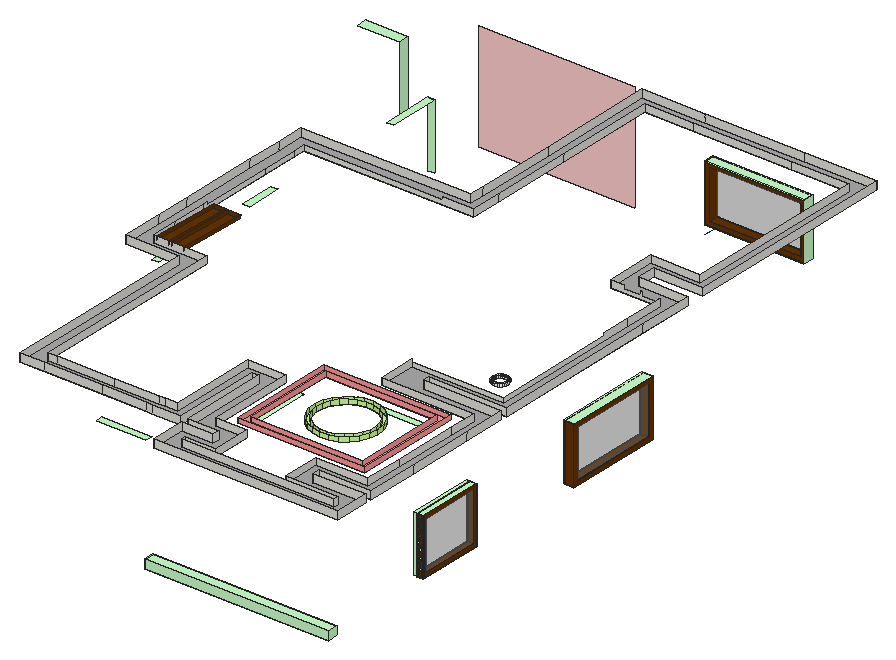
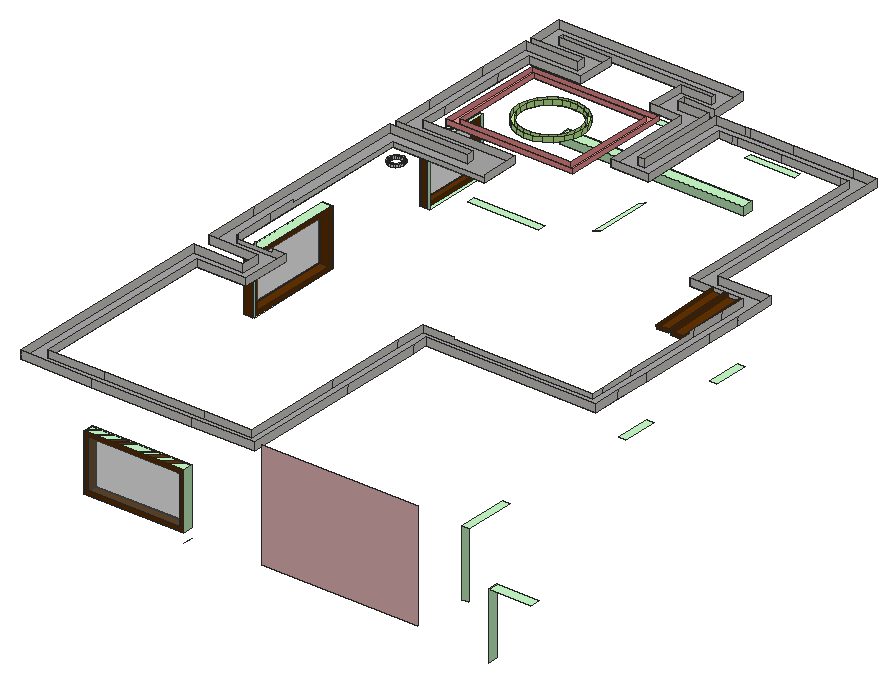
# SketchUp Ruby script. Lengths in inches.
U = 1.inch
M = Sketchup.active_model
def pt(a) = Geom::Point3d.new(a.map { |v| v * U })
def face(e, loops, mat)
  f = e.add_face(loops[0].map { |a| pt(a) })
  loops[1..].each { |l| e.add_face(l.map { |a| pt(a) }).erase! }
  f.material = f.back_material = mat if mat
  f
end
# faces: each face lists its corners as indices into pts; further lists are holes
def faces(e, pts, list, mat = nil) = list.each { |f| face(e, (f[0].is_a?(Array) ? f : [f]).map { |l| l.map { |i| pts[i] } }, mat) }
# xy, xz, yz: faces in a plane at the given z, y or x. An outline is a flat list of corners, or four numbers for a rectangle; further outlines are holes
def ring(l) = l.size == 4 ? [[l[0], l[1]], [l[2], l[1]], [l[2], l[3]], [l[0], l[3]]] : l.each_slice(2).to_a
def flat(e, list, mat, &to3) = list.each { |f| face(e, (f[0].is_a?(Array) ? f : [f]).map { |l| ring(l).map { |u, v| to3.(u, v) } }, mat) }
def xy(e, z, list, mat = nil) = flat(e, list, mat) { |x, y| [x, y, z] }
def xz(e, y, list, mat = nil) = flat(e, list, mat) { |x, z| [x, y, z] }
def yz(e, x, list, mat = nil) = flat(e, list, mat) { |y, z| [x, y, z] }
def lines(e, pts, list) = list.each { |a, b| e.add_line(pt(pts[a]), pt(pts[b])) }
# prism: a flat outline (further loops are holes) pulled along v
def prism(e, loops, v, mat = nil)
  f = face(e, loops, mat); d = Geom::Vector3d.new(v.map { |x| x * U })
  f.pushpull(f.normal.samedirection?(d) ? d.length : -d.length)
end
def box(e, o, s, mat = nil) = prism(e, [[o, [o[0] + s[0], o[1], o[2]], [o[0] + s[0], o[1] + s[1], o[2]], [o[0], o[1] + s[1], o[2]]]], [0, 0, s[2]], mat)
def at(x, y, z, deg = 0) = Geom::Transformation.translation(pt([x, y, z])) * Geom::Transformation.rotation(ORIGIN, Z_AXIS, deg.degrees)
def axes(o, x, y, z) = Geom::Transformation.new([*x, 0, *y, 0, *z, 0, *pt(o).to_a, 1])
def part(name) = M.definitions.add(name)
# library, detail: a bought-in or finely detailed component or shape, given as its bounding box
def library(name, o, s) = part(name).tap { |d| box(d.entities, o, s) }
def detail(e, o, s) = box(e.add_group.entities, o, s)
def put(e, d, t, mat = nil) = e.add_instance(d, t).tap { |i| i.material = mat if mat }
def group(e, t, mat = nil) = e.add_group.tap { |g| g.transformation = t; g.material = mat if mat }.entities
root = M.entities
M.materials.add("[Color A01]").color = [255, 204, 204]
M.materials.add("[Color A02]").color = [255, 153, 153]
M.materials.add("[Color C08]").color = [102, 51, 0]
M.materials.add("[Color F02]").color = [204, 255, 153]
M.materials.add("[Color G01]").color = [204, 255, 204]
M.materials.add("[Color M00]").color = [255, 255, 255]
M.materials.add("[Color M03]").color = [170, 170, 170]
M.materials.add("[Marble Carrara Gold Floor Tile]").color = [225, 223, 217]
M.materials.add("[Translucent Glass Gray]").color = [128, 128, 128]
M.materials["[Translucent Glass Gray]"].alpha = 0.5
c1 = part("Group\#14")
xy(c1.entities,0,[[0,0,8.11,83.5625]])
xy(c1.entities,3.3125,[[7.9,3.57,8.11,80]])
xy(c1.entities,3.3125,[[0,3.57,7.9,80]],"[Color C08]")
xy(c1.entities,44.6875,[[0,3.57,7.9,80],[7.9,3.57,8.11,80]])
xy(c1.entities,48,[[0,0,8.11,83.5625]],"[Color C08]")
xz(c1.entities,0,[[0,0,8.11,48]],"[Color C08]")
xz(c1.entities,3.57,[[7.9,3.3125,8.11,44.6875]])
xz(c1.entities,3.57,[[0,3.3125,7.9,44.6875]],"[Color C08]")
xz(c1.entities,80,[[7.9,3.3125,8.11,44.6875]])
xz(c1.entities,80,[[0,3.3125,7.9,44.6875]],"[Color C08]")
xz(c1.entities,83.5625,[[0,0,8.11,48]],"[Color C08]")
yz(c1.entities,0,[[[0,0,83.5625,48],[3.57,3.3125,80,44.6875]]],"[Color C08]")
yz(c1.entities,7.9,[[3.57,3.3125,80,44.6875]],"[Translucent Glass Gray]")
yz(c1.entities,8.11,[[[0,0,83.5625,48],[3.57,3.3125,80,44.6875]]],"[Color C08]")
box(root,[307,0,25.9375],[156,9,7],"[Color G01]")
xy(root,36,[[463,90.29,472,146.46],[463,249.52,472,333.08],[317.34,581,401.89,590]],"[Color G01]")
xy(root,84,[[463,90.29,472,146.46],[336.83,183,396.83,189],[114,248.47,120,278.47],[463,249.52,472,333.08],[114,345.1,120,375.1],
  [120,490.74,126,534.62],[22.6875,581,58.6875,590],[317.34,581,401.89,590]],"[Color G01]")
xy(root,96,[[234.6875,39,276.8125,45],[333.57,39,418.48,45]],"[Color G01]")
xy(root,113.1875,[[[307,9.4375,307,39.4375,333.57,39.4375,333.57,45.4375,307,45.4375,307,120.625,301,120.625,301,45.4375,165,45.4375,165,213.4375,120,213.4375,120,399.4375,264,399.4375,264,581.4375,463,581.4375,463,397.48,420.9375,397.48,420.9375,381.73,463,381.73,463,189.4375,396.83,189.4375,396.83,183.4375,463,183.4375,463,45.4375,418.48,45.4375,418.48,39.4375,463,39.4375,463,9.4375],[320.15,22.59,449.85,22.59,449.85,26.28,405.33,26.28,405.33,58.59,449.85,58.59,449.85,170.28,371.8,170.28,371.8,202.59,449.85,202.59,449.85,368.58,407.78,368.58,407.78,410.63,449.85,410.63,449.85,568.28,277.15,568.28,277.15,386.28,133.15,386.28,133.15,226.59,178.15,226.59,178.15,58.59,287.85,58.59,287.85,133.78,320.15,133.78,320.15,58.59,346.72,58.59,346.72,26.28,320.15,26.28]]],"[Color M03]")
xy(root,115.1875,[[[331.35,68.47,438.72,159.72],[337.55,74.67,432.52,153.52]]],"[Color A02]")
xy(root,115.1875,[[[385.83,87.07,378.78,88.18,372.26,91.07,366.71,95.54,362.51,101.31,359.95,107.96,359.1875,115.05,360.29,122.09,363.18,128.61,367.66,134.16,373.42,138.36,380.07,140.93,387.16,141.68,394.21,140.58,400.72,137.69,406.27,133.21,410.47,127.45,413.04,120.8,413.8,113.71,412.69,106.67,409.81,100.15,405.33,94.6,399.57,90.4,392.91,87.83],[388.97,90.51,395.0625,91.96,400.57,94.94,405.12,99.25,408.4,104.58,410.19,110.59,410.37,116.85,408.91,122.95,405.93,128.46,401.625,133.01,396.29,136.29,390.28,138.08,384.02,138.25,377.93,136.8,372.42,133.82,367.86,129.51,364.58,124.17,362.79,118.17,362.62,111.91,364.07,105.8125,367.06,100.3,371.36,95.75,376.7,92.47,382.7,90.68]]],"[Color F02]")
xy(root,115.1875,[[[433.35,213.79,431.59,213.8,429.89,214.26,428.36,215.15,427.125,216.4,426.25,217.93,425.8,219.63,425.81,221.4,426.27,223.1,427.16,224.62,428.41,225.86,429.94,226.74,431.64,227.19,433.4,227.18,435.1,226.72,436.625,225.83,437.87,224.58,438.74,223.05,439.19,221.35,439.18,219.58,438.72,217.88,437.83,216.36,436.58,215.12,435.05,214.24],[432.49,215.49,433.79,215.66,434.99,216.16,436.03,216.95,436.82,217.99,437.32,219.2,437.49,220.49,437.32,221.78,436.82,222.99,436.03,224.03,434.99,224.82,433.79,225.32,432.49,225.49,431.2,225.32,429.99,224.82,428.96,224.03,428.16,222.99,427.66,221.78,427.49,220.49,427.66,219.2,428.16,217.99,428.96,216.95,429.99,216.16,431.2,215.66]]],"[Color M00]")
xz(root,9.4375,[[307,113.1875,463,120]],"[Marble Carrara Gold Floor Tile]")
xz(root,22.59,[[320.15,113.1875,449.85,119.1875]],"[Marble Carrara Gold Floor Tile]")
xz(root,26.28,[[320.15,113.1875,346.72,119.1875],[405.33,113.1875,449.85,119.1875]],"[Marble Carrara Gold Floor Tile]")
xz(root,39.4375,[[307,113.1875,333.57,120],[418.48,113.1875,463,120]],"[Marble Carrara Gold Floor Tile]")
xz(root,45.4375,[[165,113.1875,185.25,120],[185.25,113.1875,234.6875,120],[234.6875,113.1875,271.8125,120],[271.8125,113.1875,276.8125,120],[276.8125,113.1875,301,120],
  [307,113.1875,333.57,120],[418.48,113.1875,463,120]],"[Marble Carrara Gold Floor Tile]")
xz(root,58.59,[[178.15,113.1875,185.25,119.1875],[185.25,113.1875,234.6875,119.1875],[234.6875,113.1875,271.8125,119.1875],[271.8125,113.1875,276.8125,119.1875],[276.8125,113.1875,287.85,119.1875],
  [320.15,113.1875,346.72,119.1875],[405.33,113.1875,449.85,119.1875]],"[Marble Carrara Gold Floor Tile]")
xz(root,68.47,[[331.35,115.1875,438.72,119.1875]],"[Color A02]")
xz(root,74.67,[[337.55,115.1875,432.52,119.1875]],"[Color A02]")
xz(root,90.29,[[463,36,472,84]],"[Color G01]")
xz(root,120.625,[[301,113.1875,307,120]],"[Marble Carrara Gold Floor Tile]")
xz(root,133.78,[[287.85,113.1875,320.15,119.1875]],"[Marble Carrara Gold Floor Tile]")
xz(root,146.46,[[463,36,472,84]],"[Color G01]")
xz(root,153.52,[[337.55,115.1875,432.52,119.1875]],"[Color A02]")
xz(root,159.72,[[331.35,115.1875,438.72,119.1875]],"[Color A02]")
xz(root,170.28,[[371.8,113.1875,449.85,119.1875]],"[Marble Carrara Gold Floor Tile]")
xz(root,183.4375,[[396.83,113.1875,463,120]],"[Marble Carrara Gold Floor Tile]")
xz(root,189.4375,[[396.83,113.1875,463,120]],"[Marble Carrara Gold Floor Tile]")
xz(root,202.59,[[371.8,113.1875,449.85,117.1875]],"[Marble Carrara Gold Floor Tile]")
xz(root,213.4375,[[120,113.1875,165,120]],"[Marble Carrara Gold Floor Tile]")
xz(root,226.59,[[133.15,113.1875,178.15,119.1875]],"[Marble Carrara Gold Floor Tile]")
xz(root,249.52,[[463,36,472,84]],"[Color G01]")
xz(root,333.08,[[463,36,472,84]],"[Color G01]")
xz(root,368.58,[[407.78,113.1875,449.85,113.1875,449.85,119.1875,448.92,119.1875,448.92,116.1875,434.49,116.1875,434.49,119.1875,433.17,119.1875,433.17,116.1875,418.74,116.1875,418.74,119.1875,407.78,119.1875]],"[Marble Carrara Gold Floor Tile]")
xz(root,381.73,[[420.9375,113.1875,463,120]],"[Marble Carrara Gold Floor Tile]")
xz(root,386.28,[[133.15,113.1875,277.15,113.1875,277.15,119.1875,251.25,119.1875,251.25,117.1875,133.15,117.1875]],"[Marble Carrara Gold Floor Tile]")
xz(root,397.48,[[420.9375,113.1875,463,120]],"[Marble Carrara Gold Floor Tile]")
xz(root,399.4375,[[120,113.1875,264,120]],"[Marble Carrara Gold Floor Tile]")
xz(root,410.63,[[407.78,113.1875,449.85,119.1875]],"[Marble Carrara Gold Floor Tile]")
xz(root,534.62,[[120,28.25,126,84]],"[Color G01]")
xz(root,568.28,[[277.15,113.1875,317.34,119.1875],[317.34,113.1875,401.89,119.1875],[401.89,113.1875,449.85,119.1875]],"[Marble Carrara Gold Floor Tile]")
xz(root,581,[[126,28.25,258,120]],"[Color A01]")
xz(root,581.4375,[[264,113.1875,317.34,120],[317.34,113.1875,401.89,120],[401.89,113.1875,463,120]],"[Marble Carrara Gold Floor Tile]")
yz(root,58.6875,[[581,28.25,590,84]],"[Color G01]")
yz(root,120,[[213.4375,113.1875,248.91,120],[248.91,113.1875,278.91,120],[278.91,113.1875,345.53,120],[345.53,113.1875,375.53,120],[375.53,113.1875,399.4375,120]],"[Marble Carrara Gold Floor Tile]")
yz(root,133.15,[[226.59,113.1875,248.91,119.1875],[248.91,113.1875,278.91,119.1875],[278.91,113.1875,345.53,113.1875,345.53,117.1875,283.41,117.1875,283.41,119.1875,278.91,119.1875],[345.53,113.1875,375.53,117.1875],[375.53,113.1875,386.28,117.1875]],"[Marble Carrara Gold Floor Tile]")
yz(root,135.92,[[287.2,114,226.48,116.1875,226.59,119.1875,287.31,116.99]],"[Color C08]")
yz(root,146.22,[[287.2,114,287.31,116.99,226.59,119.1875,226.48,116.1875]],"[Color C08]")
yz(root,148.55,[[286.58,114.02,226.48,116.1875,226.59,119.1875,286.68,117.02]],"[Color C08]")
yz(root,158.84,[[286.58,114.02,286.68,117.02,226.59,119.1875,226.48,116.1875]],"[Color C08]")
yz(root,165,[[45.4375,113.1875,213.4375,120]],"[Marble Carrara Gold Floor Tile]")
yz(root,178.15,[[58.59,113.1875,226.59,119.1875]],"[Marble Carrara Gold Floor Tile]")
yz(root,264,[[399.4375,113.1875,412.84,120],[412.84,113.1875,482.17,120],[482.17,113.1875,581.4375,120]],"[Marble Carrara Gold Floor Tile]")
yz(root,277.15,[[386.28,113.1875,412.84,119.1875],[412.84,113.1875,482.17,119.1875],[482.17,113.1875,568.28,119.1875]],"[Marble Carrara Gold Floor Tile]")
yz(root,287.85,[[58.59,113.1875,133.78,119.1875]],"[Marble Carrara Gold Floor Tile]")
yz(root,301,[[45.4375,113.1875,120.625,120]],"[Marble Carrara Gold Floor Tile]")
yz(root,307,[[9.4375,113.1875,39.4375,120],[45.4375,113.1875,120.625,120]],"[Marble Carrara Gold Floor Tile]")
yz(root,317.34,[[581,36,590,84]],"[Color G01]")
yz(root,320.15,[[22.59,113.1875,26.28,119.1875],[58.59,113.1875,133.78,119.1875]],"[Marble Carrara Gold Floor Tile]")
yz(root,331.35,[[68.47,115.1875,159.72,119.1875]],"[Color A02]")
yz(root,333.57,[[39.4375,113.1875,45.4375,120]],"[Marble Carrara Gold Floor Tile]")
yz(root,337.55,[[74.67,115.1875,153.52,119.1875]],"[Color A02]")
yz(root,346.72,[[26.28,113.1875,58.59,119.1875]],"[Marble Carrara Gold Floor Tile]")
yz(root,371.8,[[170.28,113.1875,202.59,119.1875]],"[Marble Carrara Gold Floor Tile]")
yz(root,396.83,[[183.4375,113.1875,189.4375,120]],"[Marble Carrara Gold Floor Tile]")
yz(root,401.89,[[581,36,590,84]],"[Color G01]")
yz(root,405.33,[[26.28,113.1875,58.59,119.1875]],"[Marble Carrara Gold Floor Tile]")
yz(root,407.78,[[368.58,113.1875,410.63,119.1875]],"[Marble Carrara Gold Floor Tile]")
yz(root,418.48,[[39.4375,113.1875,45.4375,120]],"[Marble Carrara Gold Floor Tile]")
yz(root,420.9375,[[381.73,113.1875,397.48,120]],"[Marble Carrara Gold Floor Tile]")
yz(root,432.52,[[74.67,115.1875,153.52,119.1875]],"[Color A02]")
yz(root,438.72,[[68.47,115.1875,159.72,119.1875]],"[Color A02]")
yz(root,449.85,[[22.59,113.1875,26.28,119.1875],[58.59,113.1875,90.72,119.1875],[90.72,113.1875,146.89,119.1875],[146.89,113.1875,170.28,119.1875],[202.59,113.1875,202.59,117.1875,309.14,117.1875,309.14,119.1875,333.52,119.1875,333.52,113.1875],
  [333.52,113.1875,368.58,119.1875],[410.63,113.1875,568.28,119.1875]],"[Marble Carrara Gold Floor Tile]")
yz(root,463,[[9.4375,113.1875,39.4375,120],[45.4375,113.1875,90.72,120],[90.72,113.1875,146.89,120],[146.89,113.1875,183.4375,120],[189.4375,113.1875,333.52,120],
  [333.52,113.1875,381.73,120],[397.48,113.1875,581.4375,120]],"[Marble Carrara Gold Floor Tile]")
p = [[301,120.1875,86.29],[301,168.1875,86.29],[307,168.1875,84],[307,120.1875,84],[307,168.3125,84],[301,168.3125,86.29],
  [135.92,226.48,116.1875],[135.92,287.2,114],[146.22,287.2,114],[146.22,226.48,116.1875],[148.55,226.48,116.1875],[148.55,286.58,114.02],
  [158.84,286.58,114.02],[158.84,226.48,116.1875],[148.55,286.68,117.02],[158.84,286.68,117.02],[135.92,287.31,116.99],[146.22,287.31,116.99],
  [385.83,87.07,119.1875],[378.78,88.18,119.1875],[378.78,88.18,115.1875],[385.83,87.07,115.1875],[392.91,87.83,119.1875],[392.91,87.83,115.1875],
  [399.57,90.4,119.1875],[399.57,90.4,115.1875],[372.26,91.07,119.1875],[372.26,91.07,115.1875],[405.33,94.6,119.1875],[405.33,94.6,115.1875],
  [382.7,90.68,119.1875],[388.97,90.51,119.1875],[388.97,90.51,115.1875],[382.7,90.68,115.1875],[395.0625,91.96,119.1875],[395.0625,91.96,115.1875],
  [376.7,92.47,119.1875],[376.7,92.47,115.1875],[366.71,95.54,119.1875],[366.71,95.54,115.1875],[400.57,94.94,119.1875],[400.57,94.94,115.1875],
  [371.36,95.75,119.1875],[371.36,95.75,115.1875],[409.81,100.15,119.1875],[409.81,100.15,115.1875],[405.12,99.25,119.1875],[405.12,99.25,115.1875],
  [362.51,101.31,119.1875],[362.51,101.31,115.1875],[367.06,100.3,119.1875],[367.06,100.3,115.1875],[408.4,104.58,119.1875],[408.4,104.58,115.1875],
  [412.69,106.67,119.1875],[412.69,106.67,115.1875],[364.07,105.8125,119.1875],[364.07,105.8125,115.1875],[359.95,107.96,119.1875],[359.95,107.96,115.1875],
  [410.19,110.59,119.1875],[410.19,110.59,115.1875],[362.62,111.91,119.1875],[362.62,111.91,115.1875],[413.8,113.71,119.1875],[413.8,113.71,115.1875],
  [359.1875,115.05,119.1875],[359.1875,115.05,115.1875],[410.37,116.85,119.1875],[410.37,116.85,115.1875],[362.79,118.17,119.1875],[362.79,118.17,115.1875],
  [413.04,120.8,119.1875],[413.04,120.8,115.1875],[360.29,122.09,119.1875],[360.29,122.09,115.1875],[408.91,122.95,119.1875],[408.91,122.95,115.1875],
  [364.58,124.17,119.1875],[364.58,124.17,115.1875],[410.47,127.45,119.1875],[410.47,127.45,115.1875],[363.18,128.61,119.1875],[363.18,128.61,115.1875],
  [405.93,128.46,119.1875],[405.93,128.46,115.1875],[367.86,129.51,119.1875],[367.86,129.51,115.1875],[406.27,133.21,119.1875],[406.27,133.21,115.1875],
  [401.625,133.01,119.1875],[401.625,133.01,115.1875],[367.66,134.16,119.1875],[367.66,134.16,115.1875],[372.42,133.82,119.1875],[372.42,133.82,115.1875],
  [396.29,136.29,119.1875],[396.29,136.29,115.1875],[400.72,137.69,119.1875],[400.72,137.69,115.1875],[377.93,136.8,119.1875],[377.93,136.8,115.1875],
  [373.42,138.36,119.1875],[373.42,138.36,115.1875],[390.28,138.08,119.1875],[390.28,138.08,115.1875],[384.02,138.25,119.1875],[384.02,138.25,115.1875],
  [394.21,140.58,119.1875],[394.21,140.58,115.1875],[380.07,140.93,119.1875],[380.07,140.93,115.1875],[387.16,141.68,119.1875],[387.16,141.68,115.1875],
  [431.59,213.8,117.1875],[429.89,214.26,117.1875],[429.89,214.26,115.1875],[431.59,213.8,115.1875],[433.35,213.79,117.1875],[433.35,213.79,115.1875],
  [435.05,214.24,117.1875],[435.05,214.24,115.1875],[436.58,215.12,117.1875],[436.58,215.12,115.1875],[428.36,215.15,117.1875],[428.36,215.15,115.1875],
  [437.83,216.36,117.1875],[437.83,216.36,115.1875],[427.125,216.4,117.1875],[427.125,216.4,115.1875],[431.2,215.66,117.1875],[432.49,215.49,117.1875],
  [432.49,215.49,115.1875],[431.2,215.66,115.1875],[433.79,215.66,117.1875],[433.79,215.66,115.1875],[429.99,216.16,117.1875],[429.99,216.16,115.1875],
  [434.99,216.16,117.1875],[434.99,216.16,115.1875],[428.96,216.95,117.1875],[428.96,216.95,115.1875],[436.03,216.95,117.1875],[436.03,216.95,115.1875],
  [426.25,217.93,117.1875],[426.25,217.93,115.1875],[438.72,217.88,117.1875],[438.72,217.88,115.1875],[428.16,217.99,117.1875],[428.16,217.99,115.1875],
  [436.82,217.99,117.1875],[436.82,217.99,115.1875],[425.8,219.63,117.1875],[425.8,219.63,115.1875],[439.18,219.58,117.1875],[439.18,219.58,115.1875],
  [427.66,219.2,117.1875],[427.66,219.2,115.1875],[437.32,219.2,117.1875],[437.32,219.2,115.1875],[427.49,220.49,117.1875],[427.49,220.49,115.1875],
  [437.49,220.49,117.1875],[437.49,220.49,115.1875],[425.81,221.4,117.1875],[425.81,221.4,115.1875],[439.19,221.35,117.1875],[439.19,221.35,115.1875],
  [427.66,221.78,117.1875],[427.66,221.78,115.1875],[437.32,221.78,117.1875],[437.32,221.78,115.1875],[438.74,223.05,117.1875],[438.74,223.05,115.1875],
  [426.27,223.1,117.1875],[426.27,223.1,115.1875],[428.16,222.99,117.1875],[428.16,222.99,115.1875],[436.82,222.99,117.1875],[436.82,222.99,115.1875],
  [428.96,224.03,117.1875],[428.96,224.03,115.1875],[436.03,224.03,117.1875],[436.03,224.03,115.1875],[437.87,224.58,117.1875],[437.87,224.58,115.1875],
  [427.16,224.62,117.1875],[427.16,224.62,115.1875],[429.99,224.82,117.1875],[429.99,224.82,115.1875],[434.99,224.82,117.1875],[434.99,224.82,115.1875],
  [428.41,225.86,117.1875],[428.41,225.86,115.1875],[436.625,225.83,117.1875],[436.625,225.83,115.1875],[431.2,225.32,117.1875],[431.2,225.32,115.1875],
  [433.79,225.32,117.1875],[433.79,225.32,115.1875],[432.49,225.49,117.1875],[432.49,225.49,115.1875],[435.1,226.72,117.1875],[435.1,226.72,115.1875],
  [429.94,226.74,117.1875],[429.94,226.74,115.1875],[431.64,227.19,117.1875],[431.64,227.19,115.1875],[433.4,227.18,117.1875],[433.4,227.18,115.1875],
  [317.34,590,28.25],[317.34,581,28.25]]
faces(root,p,[[0,1,2,3],[4,2,1,5]],"[Color G01]")
faces(root,p,[[6,7,8,9],[10,11,12,13],[14,15,12,11],[16,17,8,7]],"[Color C08]")
faces(root,p,[[18,19,20,21],[22,18,21,23],[24,22,23,25],[19,26,27,20],[28,24,25,29],[30,31,32,33],[31,34,35,32],[36,30,33,37],
  [26,38,39,27],[34,40,41,35],[42,36,37,43],[44,28,29,45],[40,46,47,41],[38,48,49,39],[50,42,43,51],[46,52,53,47],
  [54,44,45,55],[56,50,51,57],[48,58,59,49],[52,60,61,53],[62,56,57,63],[64,54,55,65],[58,66,67,59],[60,68,69,61],
  [70,62,63,71],[72,64,65,73],[66,74,75,67],[68,76,77,69],[78,70,71,79],[80,72,73,81],[74,82,83,75],[76,84,85,77],
  [86,78,79,87],[88,80,81,89],[84,90,91,85],[82,92,93,83],[94,86,87,95],[90,96,97,91],[98,88,89,99],[100,94,95,101],
  [92,102,103,93],[96,104,105,97],[106,100,101,107],[108,98,99,109],[104,106,107,105],[102,110,111,103],[112,108,109,113],[110,112,113,111]],"[Color F02]")
faces(root,p,[[114,115,116,117],[118,114,117,119],[120,118,119,121],[122,120,121,123],[115,124,125,116],[126,122,123,127],[124,128,129,125],[130,131,132,133],
  [131,134,135,132],[136,130,133,137],[134,138,139,135],[140,136,137,141],[138,142,143,139],[128,144,145,129],[146,126,127,147],[148,140,141,149],
  [142,150,151,143],[144,152,153,145],[154,146,147,155],[156,148,149,157],[150,158,159,151],[160,156,157,161],[158,162,163,159],[152,164,165,153],
  [166,154,155,167],[168,160,161,169],[162,170,171,163],[172,166,167,173],[164,174,175,165],[176,168,169,177],[170,178,179,171],[180,176,177,181],
  [178,182,183,179],[184,172,173,185],[174,186,187,175],[188,180,181,189],[182,190,191,183],[186,192,193,187],[194,184,185,195],[196,188,189,197],
  [190,198,199,191],[200,196,197,201],[198,200,201,199],[202,194,195,203],[192,204,205,193],[204,206,207,205],[208,202,203,209],[206,208,209,207]],"[Color M00]")
lines(root,p,[[210,211]])
put(root,c1,at(463.89,249.52,35.62))
put(root,c1,axes([401.74,581.89,36],[0,1,0],[-1.01,0,0],[0,0,1]))
put(root,c1,axes([466.08,90.29,36],[0.6424,0,0],[0,0.6722,0],[0,0,1]))
